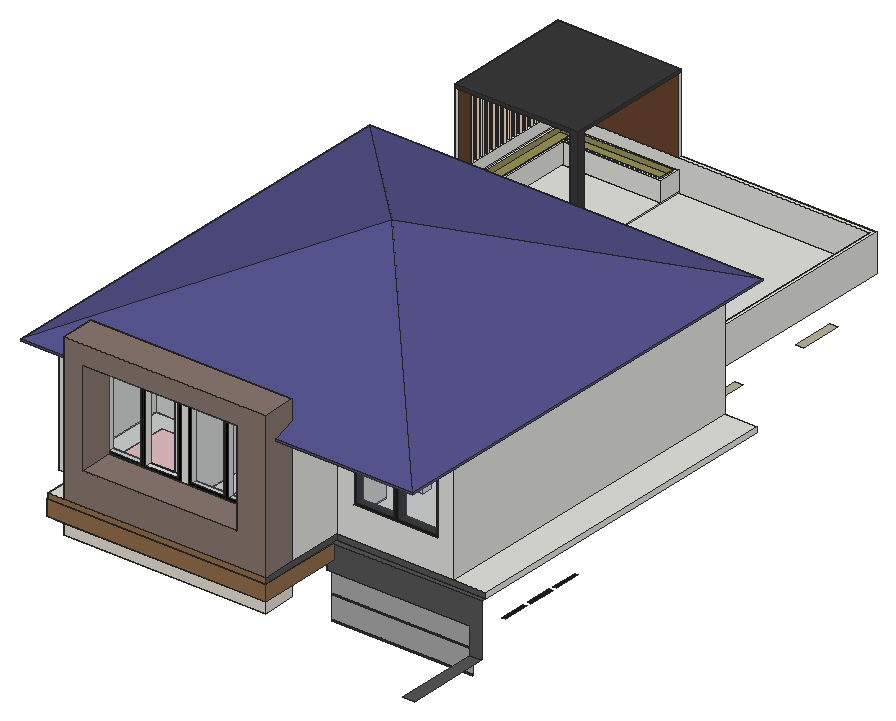
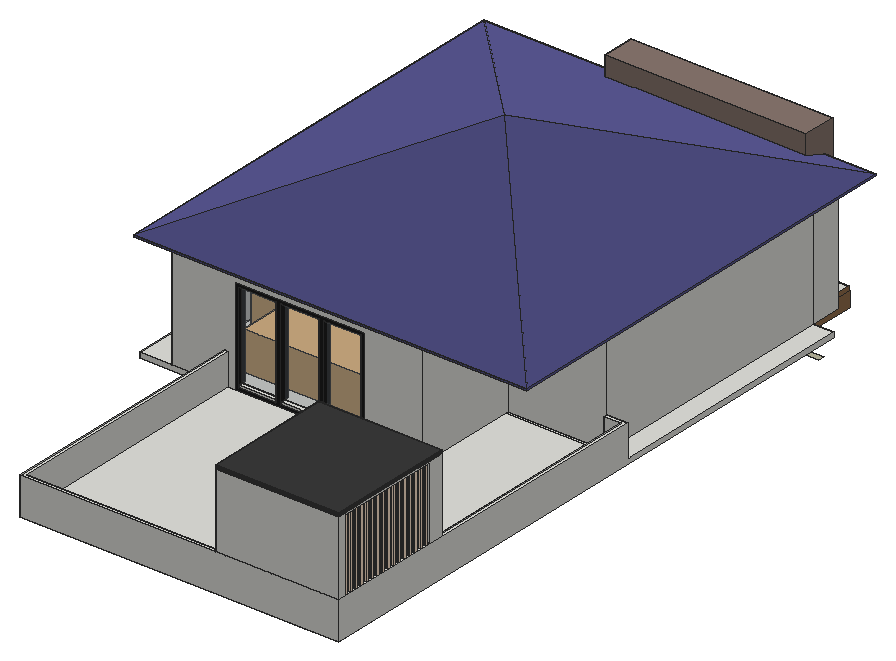
# SketchUp Ruby script. Lengths in inches.
U = 1.inch
M = Sketchup.active_model
def pt(a) = Geom::Point3d.new(a.map { |v| v * U })
def face(e, loops, mat)
  f = e.add_face(loops[0].map { |a| pt(a) })
  loops[1..].each { |l| e.add_face(l.map { |a| pt(a) }).erase! }
  f.material = f.back_material = mat if mat
  f
end
# faces: each face lists its corners as indices into pts; further lists are holes
def faces(e, pts, list, mat = nil) = list.each { |f| face(e, (f[0].is_a?(Array) ? f : [f]).map { |l| l.map { |i| pts[i] } }, mat) }
# xy, xz, yz: faces in a plane at the given z, y or x. An outline is a flat list of corners, or four numbers for a rectangle; further outlines are holes
def ring(l) = l.size == 4 ? [[l[0], l[1]], [l[2], l[1]], [l[2], l[3]], [l[0], l[3]]] : l.each_slice(2).to_a
def flat(e, list, mat, &to3) = list.each { |f| face(e, (f[0].is_a?(Array) ? f : [f]).map { |l| ring(l).map { |u, v| to3.(u, v) } }, mat) }
def xy(e, z, list, mat = nil) = flat(e, list, mat) { |x, y| [x, y, z] }
def xz(e, y, list, mat = nil) = flat(e, list, mat) { |x, z| [x, y, z] }
def yz(e, x, list, mat = nil) = flat(e, list, mat) { |y, z| [x, y, z] }
def lines(e, pts, list) = list.each { |a, b| e.add_line(pt(pts[a]), pt(pts[b])) }
# prism: a flat outline (further loops are holes) pulled along v
def prism(e, loops, v, mat = nil)
  f = face(e, loops, mat); d = Geom::Vector3d.new(v.map { |x| x * U })
  f.pushpull(f.normal.samedirection?(d) ? d.length : -d.length)
end
def box(e, o, s, mat = nil) = prism(e, [[o, [o[0] + s[0], o[1], o[2]], [o[0] + s[0], o[1] + s[1], o[2]], [o[0], o[1] + s[1], o[2]]]], [0, 0, s[2]], mat)
def at(x, y, z, deg = 0) = Geom::Transformation.translation(pt([x, y, z])) * Geom::Transformation.rotation(ORIGIN, Z_AXIS, deg.degrees)
def axes(o, x, y, z) = Geom::Transformation.new([*x, 0, *y, 0, *z, 0, *pt(o).to_a, 1])
def part(name) = M.definitions.add(name)
# library, detail: a bought-in or finely detailed component or shape, given as its bounding box
def library(name, o, s) = part(name).tap { |d| box(d.entities, o, s) }
def detail(e, o, s) = box(e.add_group.entities, o, s)
def put(e, d, t, mat = nil) = e.add_instance(d, t).tap { |i| i.material = mat if mat }
def group(e, t, mat = nil) = e.add_group.tap { |g| g.transformation = t; g.material = mat if mat }.entities
root = M.entities
M.materials.add("A01_Blush_Petal").color = [255, 204, 204]
M.materials.add("C01_Vanilla_Cream").color = [255, 230, 206]
M.materials.add("Concrete_04_1K").color = [184, 181, 156]
M.materials.add("F01_Seafoam_Drift").color = [229, 255, 204]
M.materials.add("G01_Mint_Mist").color = [204, 255, 204]
M.materials.add("Glass_Basic_01").color = [161, 173, 186]
M.materials["Glass_Basic_01"].alpha = 0.25
M.materials.add("Glass_Mirror_01").color = [185, 185, 185]
M.materials.add("L01_Cotton_Candy").color = [255, 204, 229]
M.materials.add("M03_Pewter_Shine").color = [168, 168, 168]
M.materials.add("M06_Steel_Smoke").color = [86, 86, 86]
M.materials.add("M07_Charcoal_Gleam").color = [58, 58, 58]
M.materials.add("M08_Obsidian_Black").color = [30, 30, 30]
M.materials.add("M09_Shadow_Night").color = [0, 0, 0]
M.materials.add("Marble_01_1K").color = [230, 221, 211]
M.materials.add("Metal_06_1K").color = [238, 236, 231]
M.materials.add("Plywood_08_1K").color = [202, 166, 113]
M.materials.add("Roofing_07_1K").color = [87, 85, 143]
M.materials.add("Soil_04_1K").color = [152, 146, 88]
M.materials.add("Wood_Floor_01_1K").color = [146, 111, 76]
M.materials.add("Wood_Floor_12_1K").color = [137, 119, 111]
M.materials.add("Wood_Veneer_15_1K").color = [103, 69, 45]
c1 = part("Group\#16")
box(c1.entities,[0,0,0],[9,36,9])
c2 = part("Group\#15")
box(c2.entities,[0,0,0],[9,36,9])
c3 = part("Group\#65")
detail(c3.entities,[3.98,0,0],[59.19,63.17,43.625])
c4 = library("Group\#63",[0,0,0],[138,56.37,43.625])
c5 = part("Group\#87")
prism(c5.entities,[[[12.875,15.85,0],[12.875,5.875,0],[12.54,4.32,0],[11.83,2.9,0],[10.8,1.69,0],[9.5,0.77,0],[8.02,0.2,0],[6.4375,0,0],[4.86,0.2,0],[3.375,0.77,0],[2.08,1.69,0],[1.05,2.9,0],[0.34,4.32,0],[0,5.875,0],[0,15.85,0],[0.52,17.21,0],[1.32,18.43,0],[2.37,19.44,0],[3.61,20.2,0],[4.99,20.67,0],[6.4375,20.83,0],[7.89,20.67,0],[9.27,20.2,0],[10.51,19.44,0],[11.56,18.43,0],[12.36,17.21,0]]],[0,0,2])
c6 = part("Group\#86")
xy(c6.entities,0,[[0,0,78.6875,56.125]])
xy(c6.entities,12,[[0,0,78.6875,56.125]],"A01_Blush_Petal")
xz(c6.entities,0,[[0,0,78.6875,12]],"A01_Blush_Petal")
xz(c6.entities,56.125,[[0,0,78.6875,12]],"A01_Blush_Petal")
yz(c6.entities,0,[[0,0,56.125,12]])
yz(c6.entities,78.6875,[[0,0,56.125,12]],"A01_Blush_Petal")
put(c6.entities,c5,at(5.56,5.57,12),"G01_Mint_Mist")
put(c6.entities,c5,at(5.56,28.95,12),"G01_Mint_Mist")
xy(root,81.29,[[4861.07,3566.51,4874.8125,3660.98]],"M06_Steel_Smoke")
xy(root,99,[[4550.5625,3805.79,4586.5625,3809.79],[4591.8125,3833.04,4595.8125,3869.04],[4784.8125,3923.04,4825.3125,3929.04],[4586.8125,4226.61,4591.8125,4262.61]],"Concrete_04_1K")
xy(root,105.07,[[4586.8125,3932.41,4591.3125,3997.24],[4591.3125,3932.41,4595.8125,3997.24]],"M08_Obsidian_Black")
xy(root,107.45,[[4584.8125,4077.51,4588.3125,4117.75],[4588.3125,4077.51,4591.8125,4117.75],[4584.8125,4127.84,4588.3125,4177.75],[4588.3125,4127.84,4591.8125,4177.75]],"M08_Obsidian_Black")
xy(root,108,[[4870.8125,3694.73,4874.8125,3724.73],[4870.8125,3730.73,4874.8125,3760.73],[4870.8125,3766.73,4874.8125,3796.73],[4492.8125,4193.04,4518.8125,4197.54],[4520.8125,4193.04,4546.8125,4197.54]],"M08_Obsidian_Black")
xy(root,111,[[4498.625,3604.45,4546.625,3606.54],[4553.37,3604.45,4601.37,3608.64],[4498.625,3606.54,4546.625,3608.64],[4634.06,3666.98,4682.06,3670.98],[4769.8125,4101.42,4778.8125,4149.42],
  [4489.8125,4193.04,4549.8125,4197.54],[4489.8125,4197.54,4549.8125,4202.04],[4769.8125,4234.61,4778.8125,4282.61]],"Concrete_04_1K")
xy(root,111,[[4700.3125,3660.98,4861.07,3666.98]],"M06_Steel_Smoke")
xy(root,111,[[4584.8125,4073.96,4586.8125,4121.29],[4584.8125,4124.29,4586.8125,4181.29]],"M08_Obsidian_Black")
xy(root,117.5625,[[4432.07,3639.11,4462.07,3645.11]],"Concrete_04_1K")
xy(root,124.125,[[4462.07,3564.51,4480,3639.11]],"Concrete_04_1K")
xy(root,124.125,[[4480,3564.51,4480,3604.45,4700.3125,3604.45,4700.3125,3660.98,4708.6875,3660.98,4708.6875,3564.51]],"Plywood_08_1K")
xy(root,141,[[[4480,3604.45,4625.87,3604.45,4625.87,3666.98,4695.7,3666.98,4695.7,3604.45,4700.3125,3604.45,4700.3125,3666.98,4874.8125,3666.98,4874.8125,3833.04,4870.8125,3833.04,4870.8125,3670.98,4690.8125,3670.98,4690.8125,3833.04,4686.8125,3833.04,4686.8125,3670.98,4625.87,3670.98,4625.87,3750.01,4595.8125,3750.01,4595.8125,3878.04,4480,3878.04,4480,3809.79,4420.38,3809.79,4420.38,3639.11,4480,3639.11],[4489,3608.64,4489,3805.79,4591.8125,3805.79,4591.8125,3746.01,4621.87,3746.01,4621.87,3608.64],[4429.38,3645.11,4480,3800.79],[4489,3809.79,4591.8125,3869.04]],[4646.8125,3770.04,4650.8125,3770.04,4650.8125,3869.04,4741.125,3869.04,4741.125,3878.04,4646.8125,3878.04],[4690.8125,3829.04,4741.125,3833.04],[4777.125,3829.04,4870.8125,3833.04],[[4865.8125,3833.04,4874.8125,3833.04,4874.8125,4049.04,4778.8125,4049.04,4778.8125,4337.04,4454.8125,4337.04,4454.8125,4193.04,4586.8125,4193.04,4586.8125,4058.04,4480,4058.04,4480,4049.04,4591.8125,4049.04,4591.8125,4328.04,4769.8125,4328.04,4769.8125,4040.04,4865.8125,4040.04,4865.8125,3983.04,4784.8125,3983.04,4784.8125,4010.04,4778.8125,4010.04,4778.8125,3869.04,4784.8125,3869.04,4784.8125,3923.04,4825.3125,3923.04,4825.3125,3929.04,4784.8125,3929.04,4784.8125,3977.04,4865.8125,3977.04,4865.8125,3929.04,4825.3125,3929.04,4825.3125,3923.04,4865.8125,3923.04],[4463.8125,4202.04,4586.8125,4328.04]],
  [4586.8125,3878.04,4595.8125,4049.04],[4708.76,3915.92,4736.64,3915.92,4736.64,4049.04,4708.76,4049.04,4708.76,4045.04,4732.01,4045.04,4732.01,3919.92,4708.76,3919.92]],"Concrete_04_1K")
xy(root,141,[[4700.3125,3604.45,4708.6875,3604.45,4708.6875,3660.98,4874.8125,3660.98,4874.8125,3666.98,4700.3125,3666.98]],"M06_Steel_Smoke")
xy(root,141.1875,[[4462.07,3564.51,4708.6875,3564.51,4708.6875,3604.45,4480,3604.45,4480,3639.11,4462.07,3639.11]],"Wood_Floor_01_1K")
xy(root,153,[[4612.42,3619.02,4666.3,3697.33],[4489.57,3621.3125,4540.88,3691.6875]])
xz(root,3564.51,[[4462.07,124.125,4708.6875,141.1875]],"Wood_Floor_01_1K")
xz(root,3604.45,[[4480,124.125,4625.87,141],[4625.87,124.125,4695.7,141],[4695.7,124.125,4700.3125,141],[4480,141,4700.3125,141.1875],[4700.3125,141,4708.6875,141.1875]],"Concrete_04_1K")
xz(root,3639.11,[[4462.07,124.125,4480,141],[4462.07,141,4480,141.1875]],"Concrete_04_1K")
xz(root,3660.98,[[4861.07,81.29,4874.8125,81.29,4874.8125,141,4708.6875,141,4708.6875,124.125,4700.3125,124.125,4700.3125,111,4861.07,111]],"M06_Steel_Smoke")
xz(root,3666.98,[[4701.3125,60,4860.07,84],[4701.3125,86,4860.07,110]],"M03_Pewter_Shine")
xz(root,3666.98,[[4701.3125,58,4860.07,60],[4701.3125,84,4860.07,86]],"M07_Charcoal_Gleam")
xz(root,3923.04,[[4784.8125,99,4825.3125,141]],"M03_Pewter_Shine")
xz(root,3929.04,[[4784.8125,99,4825.3125,141]],"L01_Cotton_Candy")
yz(root,4462.07,[[3564.51,124.125,3639.11,141.1875]],"Wood_Floor_01_1K")
yz(root,4480,[[3604.45,124.125,3639.11,141],[3604.45,141,3639.11,141.1875]],"Concrete_04_1K")
yz(root,4591.8125,[[3833.04,99,3869.04,141]],"L01_Cotton_Candy")
yz(root,4595.8125,[[3833.04,99,3869.04,141]],"L01_Cotton_Candy")
yz(root,4700.3125,[[3660.98,111,3666.98,111,3666.98,141,3604.45,141,3604.45,124.125,3660.98,124.125]],"Concrete_04_1K")
yz(root,4708.6875,[[3564.51,124.125,3660.98,124.125,3660.98,141,3604.45,141,3604.45,141.1875,3564.51,141.1875]],"Wood_Floor_01_1K")
g1 = group(root,at(4578.37,3805.79,56.68))
prism(g1,[[[1.19,0,3.08],[1.59,0,3.125],[1.99,0,3.0625],[2.37,0,2.9],[2.6875,0,2.65],[2.93,0,2.32],[3.08,0,1.9375],[3.125,0,1.53],[3.0625,0,1.13],[2.9,0,0.76],[2.65,0,0.4375],[2.32,0,0.2],[1.9375,0,0.05],[1.53,0,0],[1.13,0,0.0625],[0.76,0,0.22],[0.4375,0,0.48],[0.2,0,0.81],[0.05,0,1.19],[0,0,1.59],[0.0625,0,1.99],[0.22,0,2.37],[0.48,0,2.6875],[0.81,0,2.93]]],[0,-0.4375,0],"Metal_06_1K")
g2 = group(root,at(4521.09,3785.04,69.49))
prism(g2,[[[1.39,0,3.6875],[1.875,0,3.75],[2.36,0,3.6875],[2.8125,0,3.5],[3.2,0,3.2],[3.5,0,2.8125],[3.6875,0,2.36],[3.75,0,1.875],[3.6875,0,1.39],[3.5,0,0.9375],[3.2,0,0.55],[2.8125,0,0.25],[2.36,0,0.0625],[1.875,0,0],[1.39,0,0.0625],[0.9375,0,0.25],[0.55,0,0.55],[0.25,0,0.9375],[0.0625,0,1.39],[0,0,1.875],[0.0625,0,2.36],[0.25,0,2.8125],[0.55,0,3.2],[0.9375,0,3.5]]],[0,-1,0],"Metal_06_1K")
g3 = group(root,at(4480,3604.45,111))
box(g3,[0,-37.9375,0],[226.6875,37.9375,13.125],"Marble_01_1K")
g4 = group(root,at(4443.375,3604.44,141))
xy(g4,0,[[234.125,264.6,240.125,273.6],[240.125,264.6,289.8125,273.6]])
xy(g4,6,[[161.8125,165.6,197.8125,174.6],[161.8125,174.6,197.8125,183.6],[161.8125,183.6,197.8125,192.6],[161.8125,192.6,197.8125,201.6],[161.8125,201.6,197.8125,210.6],
  [161.8125,210.6,197.8125,219.6],[161.8125,219.6,197.8125,228.6],[161.8125,228.6,197.8125,264.6],[197.8125,228.6,207.125,264.6],[207.125,228.6,216.125,264.6],
  [216.125,228.6,225.125,264.6],[225.125,228.6,234.125,264.6],[234.125,228.6,243.125,264.6],[243.125,228.6,252.125,264.6],[252.125,228.6,289.8125,264.6]])
xz(g4,228.6,[[197.8125,0,201.8125,6],[201.8125,0,289.8125,6]])
xz(g4,264.6,[[234.125,0,240.125,6],[240.125,0,289.8125,6]])
xz(g4,273.6,[[234.125,0,240.125,6],[240.125,0,289.8125,6]])
yz(g4,289.8125,[[228.6,0,264.6,6],[264.6,0,273.6,6]])
g5 = group(g4,at(0,0,6))
xy(g5,0,[[[0,0,0,325.35,111.8125,325.35,111.8125,444.6,394.8125,444.6,394.8125,62.54,263.3125,62.54,263.3125,0],[9,6,125.66,6,125.66,132,218.3125,132,218.3125,126,131.66,126,131.66,6,254.3125,6,254.3125,132,263.3125,132,263.3125,71.54,385.8125,71.54,385.8125,435.6,174.8125,435.6,174.8125,393.6,120.8125,393.6,120.8125,196.35,111.8125,196.35,111.8125,316.35,9,316.35,9,205.35,75.8125,205.35,75.8125,188.61,69.8125,188.61,69.8125,196.35,9,196.35,9,132,69.8125,132,69.8125,158.61,75.8125,158.61,75.8125,132,89.66,132,89.66,126,9,126],[120.8125,399.6,168.8125,435.6]]])
xy(g5,3,[[181.875,435.6,223.67,444.6],[229.67,435.6,271.875,444.6],[277.875,435.6,319.875,444.6]])
xy(g5,6,[[9,6,125.66,126],[131.66,6,254.3125,126],[[263.3125,71.54,385.8125,71.54,385.8125,435.6,319.875,435.6,319.875,440.1,277.875,440.1,277.875,435.6,271.875,435.6,271.875,440.1,229.67,440.1,229.67,435.6,223.67,435.6,223.67,440.1,181.875,440.1,181.875,435.6,174.8125,435.6,174.8125,393.6,120.8125,393.6,120.8125,196.35,75.8125,196.35,75.8125,132,263.3125,132],[197.8125,158.6,197.8125,165.6,157.8125,165.6,157.8125,268.6,234.125,268.6,234.125,273.6,289.8125,273.6,289.8125,228.6,283.8125,228.6,283.8125,199.98,277.8125,199.98,277.8125,169.98,283.8125,169.98,283.8125,158.6]],[89.66,126,125.66,132],[218.3125,126,254.3125,132],
  [9,132,69.8125,196.35],[69.8125,158.61,75.8125,188.61],[197.8125,164.6,197.8125,228.6,283.8125,228.6,283.8125,222.6,203.8125,222.6,203.8125,164.6],[203.8125,164.6,277.8125,222.6],[157.8125,165.6,161.8125,268.6],
  [161.8125,165.6,197.8125,174.6],[161.8125,174.6,197.8125,183.6],[161.8125,183.6,197.8125,192.6],[161.8125,192.6,197.8125,201.6],[75.8125,196.35,111.8125,205.35],
  [161.8125,201.6,197.8125,210.6],[9,205.35,111.8125,316.35],[161.8125,210.6,197.8125,219.6],[161.8125,219.6,197.8125,228.6],[161.8125,228.6,197.8125,264.6],
  [197.8125,228.6,207.125,264.6],[207.125,228.6,216.125,264.6],[216.125,228.6,225.125,264.6],[225.125,228.6,234.125,264.6],[234.125,228.6,243.125,264.6],
  [252.125,228.6,289.8125,264.6],[120.8125,399.6,168.8125,435.6],[223.67,435.6,229.67,440.1],[271.875,435.6,277.875,440.1],[181.875,440.1,223.67,444.6],
  [229.67,440.1,271.875,444.6],[277.875,440.1,319.875,444.6]])
xy(g5,39,[[20.75,0,50.75,6],[56.75,0,92.75,6],[98.75,0,134.75,6],[149.625,0,185.625,6],[191.625,0,227.625,6]])
xy(g5,39,[[285.75,62.54,327.75,71.54],[333.75,62.54,375.75,71.54]],"M08_Obsidian_Black")
xy(g5,90,[[277.8125,169.98,283.8125,199.98]])
xy(g5,105,[[181.875,435.6,223.67,440.1],[229.67,435.6,271.875,440.1],[277.875,435.6,319.875,440.1],[181.875,440.1,223.67,444.6],[229.67,440.1,271.875,444.6],
  [277.875,440.1,319.875,444.6]])
xy(g5,126.25,[[20.75,0,50.75,6],[56.75,0,92.75,6],[98.75,0,134.75,6],[149.625,0,185.625,6],[191.625,0,227.625,6]])
xy(g5,126.6875,[[285.75,62.54,327.75,71.54],[333.75,62.54,375.75,71.54]],"M08_Obsidian_Black")
xy(g5,132,[[[0,0,263.3125,0,263.3125,62.54,394.8125,62.54,394.8125,444.6,111.8125,444.6,111.8125,325.35,0,325.35],[9,6,9,126,89.66,126,89.66,132,75.8125,132,75.8125,158.61,69.8125,158.61,69.8125,132,9,132,9,196.35,69.8125,196.35,69.8125,188.61,75.8125,188.61,75.8125,205.35,9,205.35,9,316.35,111.8125,316.35,111.8125,196.35,120.8125,196.35,120.8125,393.6,174.8125,393.6,174.8125,435.6,385.8125,435.6,385.8125,71.54,263.3125,71.54,263.3125,132,254.3125,132,254.3125,6,131.66,6,131.66,126,218.3125,126,218.3125,132,125.66,132,125.66,6],[120.8125,399.6,168.8125,435.6]],[197.8125,158.6,283.8125,158.6,283.8125,222.6,277.8125,222.6,277.8125,164.6,197.8125,164.6],[197.8125,164.6,203.8125,164.6,203.8125,222.6,283.8125,222.6,283.8125,228.6,197.8125,228.6]])
xy(g5,133.875,[[157.8125,165.6,161.8125,268.6],[161.8125,264.6,289.8125,264.6,289.8125,273.6,234.125,273.6,234.125,268.6,161.8125,268.6]])
xz(g5,0,[[[0,0,263.3125,132],[17.75,36,137.75,129.25],[146.625,36,230.625,129.25]]])
xz(g5,0,[[20.75,39,50.75,126.25],[56.75,39,92.75,126.25],[149.625,39,185.625,126.25],[191.625,39,227.625,126.25]],"Glass_Basic_01")
xz(g5,0,[[[17.75,36,53.75,129.25],[20.75,39,50.75,126.25]],[[53.75,36,95.75,129.25],[56.75,39,92.75,126.25]],[[95.75,36,137.75,129.25],[98.75,39,134.75,126.25]],[[146.625,36,188.625,129.25],[149.625,39,185.625,126.25]],[[188.625,36,230.625,129.25],[191.625,39,227.625,126.25]]],"M09_Shadow_Night")
xz(g5,6,[[9,0,125.66,6],[131.66,0,254.3125,6],[[9,6,9,132,125.66,132,125.66,126.25,98.75,126.25,98.75,39,125.66,39,125.66,6],[56.75,39,92.75,126.25],[20.75,39,50.75,126.25]],[[131.66,6,131.66,39,134.75,39,134.75,126.25,131.66,126.25,131.66,132,254.3125,132,254.3125,6],[149.625,39,185.625,126.25],[191.625,39,227.625,126.25]],[125.66,39,131.66,126.25],
  [131.66,39,134.75,126.25]])
xz(g5,6,[[98.75,39,125.66,126.25]],"Glass_Basic_01")
xz(g5,62.54,[[[263.3125,0,394.8125,132],[282.75,36,378.75,129.6875]]])
xz(g5,62.54,[[[282.75,36,378.75,129.6875],[285.75,39,327.75,126.6875],[333.75,39,375.75,126.6875]]],"M08_Obsidian_Black")
xz(g5,71.54,[[263.3125,0,385.8125,6],[[263.3125,6,385.8125,132],[285.75,39,327.75,126.6875],[333.75,39,375.75,126.6875]]])
xz(g5,126,[[9,0,89.66,6],[131.66,0,218.3125,6],[9,6,89.66,132],[131.66,6,218.3125,132]])
xz(g5,132,[[9,0,69.8125,6],[75.8125,0,81,6],[81,0,87,6],[87,0,89.66,6],[125.66,0,218.3125,6],
  [254.3125,0,263.3125,6],[9,6,69.8125,132],[75.8125,6,81,132],[81,6,87,132],[87,6,89.66,132],
  [125.66,6,218.3125,132],[254.3125,6,263.3125,132]])
xz(g5,158.6,[[197.8125,6,283.8125,132]])
xz(g5,158.61,[[69.8125,0,75.8125,6],[69.8125,6,75.8125,132]])
xz(g5,164.6,[[197.8125,6,203.8125,132],[203.8125,6,277.8125,132]])
xz(g5,165.6,[[157.8125,6,161.8125,133.875]])
xz(g5,169.98,[[277.8125,6,283.8125,90]])
xz(g5,188.61,[[69.8125,0,75.8125,6],[69.8125,6,75.8125,132]])
xz(g5,196.35,[[9,0,69.8125,6],[111.8125,0,120.8125,6],[9,6,69.8125,132],[111.8125,6,120.8125,132]])
xz(g5,199.98,[[277.8125,6,283.8125,90]])
xz(g5,205.35,[[9,0,75.8125,6],[9,6,75.8125,132]])
xz(g5,222.6,[[203.8125,6,277.8125,132],[277.8125,6,283.8125,132]])
xz(g5,228.6,[[197.8125,6,283.8125,132]])
xz(g5,264.6,[[161.8125,6,243.125,133.875],[243.125,6,252.125,133.875],[252.125,6,289.8125,133.875]])
xz(g5,268.6,[[157.8125,6,161.8125,133.875],[161.8125,6,234.125,133.875]])
xz(g5,273.6,[[234.125,6,289.8125,133.875]])
xz(g5,316.35,[[9,0,111.8125,6],[9,6,111.8125,132]])
xz(g5,325.35,[[0,0,111.8125,132]])
xz(g5,393.6,[[120.8125,0,174.8125,6],[120.8125,6,174.8125,132]])
xz(g5,399.6,[[120.8125,0,168.8125,6],[120.8125,6,168.8125,132]])
xz(g5,435.6,[[120.8125,0,168.8125,6],[174.8125,0,385.8125,0,385.8125,6,319.875,6,319.875,3,277.875,3,277.875,6,271.875,6,271.875,3,229.67,3,229.67,6,223.67,6,223.67,3,181.875,3,181.875,6,174.8125,6],[120.8125,6,168.8125,132],[174.8125,6,181.875,6,181.875,105,223.67,105,223.67,6,229.67,6,229.67,105,271.875,105,271.875,6,277.875,6,277.875,105,319.875,105,319.875,6,385.8125,6,385.8125,132,174.8125,132]])
xz(g5,444.6,[[111.8125,0,111.8125,132,394.8125,132,394.8125,0,322.875,0,322.875,108,178.875,108,178.875,0],[181.875,3,223.67,6],[229.67,3,271.875,6],[277.875,3,319.875,6]])
xz(g5,444.6,[[[178.875,0,322.875,108],[229.67,3,271.875,105],[277.875,3,319.875,105],[181.875,3,223.67,105]]],"M08_Obsidian_Black")
yz(g5,0,[[0,0,34.67,132],[34.67,0,325.35,132]])
yz(g5,9,[[6,0,126,6],[132,0,196.35,6],[205.35,0,316.35,6],[6,6,126,132],[132,6,196.35,132],
  [205.35,6,316.35,132]])
yz(g5,20.75,[[0,39,6,126.25]])
yz(g5,50.75,[[0,39,6,126.25]])
yz(g5,56.75,[[0,39,6,126.25]])
yz(g5,69.8125,[[132,0,158.61,6],[188.61,0,196.35,6],[132,6,158.61,132],[188.61,6,196.35,132]])
yz(g5,75.8125,[[132,0,158.61,6],[188.61,0,196.35,6],[196.35,0,205.35,6],[132,6,158.61,132],[188.61,6,196.35,132],
  [196.35,6,205.35,132]])
yz(g5,89.66,[[126,0,132,6],[126,6,132,132]])
yz(g5,92.75,[[0,39,6,126.25]])
yz(g5,98.75,[[0,39,6,126.25]])
yz(g5,111.8125,[[196.35,0,205.35,6],[205.35,0,316.35,6],[325.35,0,444.6,132],[196.35,6,205.35,132],[205.35,6,316.35,132]])
yz(g5,120.8125,[[196.35,0,393.6,6],[399.6,0,435.6,6],[196.35,6,393.6,132],[399.6,6,435.6,132]])
yz(g5,125.66,[[6,0,126,6],[126,0,132,6],[6,6,126,132],[126,6,132,132]])
yz(g5,131.66,[[6,0,126,6],[6,6,126,132]])
yz(g5,134.75,[[0,39,6,126.25]])
yz(g5,149.625,[[0,39,6,126.25]])
yz(g5,157.8125,[[165.6,6,268.6,133.875]])
yz(g5,161.8125,[[165.6,6,264.6,133.875],[264.6,6,268.6,133.875]])
yz(g5,168.8125,[[399.6,0,435.6,6],[399.6,6,435.6,132]])
yz(g5,174.8125,[[393.6,0,435.6,6],[393.6,6,435.6,132]])
yz(g5,181.875,[[435.6,3,444.6,6]])
yz(g5,181.875,[[435.6,6,440.1,105],[440.1,6,444.6,105]],"M08_Obsidian_Black")
yz(g5,185.625,[[0,39,6,126.25]])
yz(g5,191.625,[[0,39,6,126.25]])
yz(g5,197.8125,[[158.6,6,164.6,132],[164.6,6,174.6,132],[174.6,6,228.6,132]])
yz(g5,203.8125,[[164.6,6,222.6,132]])
yz(g5,218.3125,[[126,0,132,6],[126,6,132,132]])
yz(g5,223.67,[[435.6,3,444.6,6]])
yz(g5,223.67,[[435.6,6,444.6,105]],"M08_Obsidian_Black")
yz(g5,227.625,[[0,39,6,126.25]])
yz(g5,229.67,[[435.6,3,444.6,6]])
yz(g5,229.67,[[435.6,6,444.6,105]],"M08_Obsidian_Black")
yz(g5,234.125,[[268.6,6,273.6,133.875]])
yz(g5,254.3125,[[6,0,126,6],[126,0,132,6],[6,6,126,132],[126,6,132,132]])
yz(g5,263.3125,[[0,0,62.54,132],[71.54,0,132,6],[71.54,6,132,132]])
yz(g5,271.875,[[435.6,3,444.6,6]])
yz(g5,271.875,[[435.6,6,444.6,105]],"M08_Obsidian_Black")
yz(g5,277.8125,[[164.6,6,164.6,132,222.6,132,222.6,6,199.98,6,199.98,90,169.98,90,169.98,6]])
yz(g5,277.875,[[435.6,3,444.6,6]])
yz(g5,277.875,[[435.6,6,444.6,105]],"M08_Obsidian_Black")
yz(g5,283.8125,[[158.6,6,169.98,6,169.98,90,199.98,90,199.98,6,222.6,6,222.6,132,158.6,132],[222.6,6,228.6,132]])
yz(g5,285.75,[[62.54,39,71.54,126.6875]],"M08_Obsidian_Black")
yz(g5,289.8125,[[264.6,6,273.6,133.875]])
yz(g5,319.875,[[435.6,3,444.6,6]])
yz(g5,319.875,[[435.6,6,440.1,105],[440.1,6,444.6,105]],"M08_Obsidian_Black")
yz(g5,327.75,[[62.54,39,71.54,126.6875]],"M08_Obsidian_Black")
yz(g5,333.75,[[62.54,39,71.54,126.6875]],"M08_Obsidian_Black")
yz(g5,375.75,[[62.54,39,71.54,126.6875]],"M08_Obsidian_Black")
yz(g5,385.8125,[[71.54,0,435.6,6],[71.54,6,435.6,132]])
yz(g5,394.8125,[[62.54,0,444.6,132]])
p = [[197.8125,165.6,0],[197.8125,152.6,0],[265.625,152.6,0],[289.8125,152.6,0],[289.8125,228.6,0],[289.8125,191.84,0],
  [234.125,268.6,0],[157.8125,268.6,0],[157.8125,165.6,0],[161.8125,165.6,0],[289.8125,161.84,0],[283.8125,161.84,0],
  [283.8125,191.84,0]]
lines(g5,p,[[0,1],[1,2],[2,3],[4,5],[6,7],[7,8],[9,8],[10,3],[11,10],[5,10],[12,5]])
put(g5,c1,at(243.125,228.6,6))
put(g5,c1,at(234.125,228.6,15))
put(g5,c1,at(225.125,228.6,24))
put(g5,c1,at(216.125,228.6,33))
put(g5,c1,at(207.125,228.6,42))
put(g5,c1,at(198.125,228.6,51))
g6 = group(g5,at(189.125,228.6,60))
box(g6,[-27.3125,0,0],[36.3125,36,9])
put(g5,c2,at(198.125,219.6,69,90))
put(g5,c2,at(198.125,210.6,78,90))
put(g5,c2,at(198.125,201.6,87,90))
put(g5,c2,at(198.125,192.6,96,90))
put(g5,c2,at(198.125,183.6,105,90))
put(g5,c2,at(198.125,174.6,114,90))
put(g5,c2,at(198.125,165.6,123,90))
g7 = group(g5,at(181.875,440.1,6),"Glass_Basic_01")
xz(g7,0,[[0,0,138,99]])
g8 = group(root,at(4454.8125,3666.98,141))
xy(g8,0,[[7.26,-100.47,7.26,-27.875,-34.43,-27.875,-34.43,670.0625,324,670.0625,324,382.0625,420,382.0625,420,0,251.875,0,251.875,-100.47]])
xy(g8,6,[[7.26,-100.47,251.875,-100.47,251.875,0,420,0,420,382.0625,320,382.0625,320,666.0625,-30.43,666.0625,-30.43,266.8125,100.375,266.8125,100.375,262.8125,-34.43,262.8125,-34.43,-27.875,7.26,-27.875],[-11.4375,262.8125,100.375,266.8125]])
xy(g8,42,[[-34.43,262.8125,-11.4375,262.8125,-11.4375,266.8125,-30.43,266.8125,-30.43,524.58,-34.43,524.58],[320,382.0625,324,382.0625,324,670.0625,104.06,670.0625,104.06,666.0625,320,666.0625],[-34.43,524.58,-30.43,540.68],[-34.43,540.68,-30.43,661.0625],[-34.43,661.0625,-34.43,670.0625,104.06,670.0625,104.06,666.0625,-30.43,666.0625,-30.43,661.0625]])
xy(g8,123.57,[[-34.43,540.68,-30.43,661.0625]])
xy(g8,126,[[-34.43,524.58,-30.43,666.0625],[-34.43,666.0625,104.06,670.0625]])
xz(g8,-100.47,[[7.26,0,251.875,6]],"Wood_Floor_01_1K")
xz(g8,-27.875,[[-34.43,0,7.26,6]])
xz(g8,0,[[251.875,0,420,6]],"M06_Steel_Smoke")
xz(g8,262.8125,[[-34.43,6,-11.4375,42]])
xz(g8,266.8125,[[-30.43,6,-11.4375,42]])
xz(g8,382.0625,[[324,0,420,6],[320,6,324,42]])
xz(g8,524.58,[[-34.43,42,-30.43,126]])
xz(g8,540.68,[[-34.43,42,-30.43,123.57]])
xz(g8,661.0625,[[-34.43,42,-30.43,123.57]])
xz(g8,666.0625,[[-30.43,6,320,42]])
xz(g8,666.0625,[[-30.43,42,104.06,126]],"Wood_Veneer_15_1K")
xz(g8,670.0625,[[-34.43,0,324,42],[-34.43,42,104.06,126]])
yz(g8,-34.43,[[-27.875,0,-27.875,6,262.8125,6,262.8125,42,670.0625,42,670.0625,0],[524.58,42,524.58,126,670.0625,126,670.0625,42,661.0625,42,661.0625,123.57,540.68,123.57,540.68,42]])
yz(g8,-30.43,[[266.8125,6,666.0625,42]])
yz(g8,-30.43,[[524.58,42,540.68,42,540.68,123.57,661.0625,123.57,661.0625,42,666.0625,42,666.0625,126,524.58,126]],"Wood_Veneer_15_1K")
yz(g8,-11.4375,[[262.8125,6,266.8125,42]])
yz(g8,7.26,[[-100.47,0,-27.875,6]],"Wood_Floor_01_1K")
yz(g8,104.06,[[666.0625,42,670.0625,126]])
yz(g8,251.875,[[-100.47,0,0,6]],"M06_Steel_Smoke")
yz(g8,320,[[382.0625,6,666.0625,42]])
yz(g8,324,[[382.0625,0,670.0625,42]])
yz(g8,420,[[0,0,382.0625,6]])
p = [[0,526.0625,0],[-34.43,526.0625,0]]
lines(g8,p,[[0,1]])
g9 = group(g8,at(-30.43,524.58,6))
box(g9,[0,0,0],[134.49,141.49,1])
g10 = group(g8,at(-30.43,524.58,126),"M07_Charcoal_Gleam")
xy(g10,-120,[[125.49,0,134.49,9]])
xy(g10,0,[[-4,0,-4,145.49,134.49,145.49,134.49,9,125.49,9,125.49,0]])
xy(g10,4,[[-4,0,134.49,145.49]])
xz(g10,0,[[125.49,-120,134.49,-120,134.49,4,-4,4,-4,0,125.49,0]])
xz(g10,9,[[125.49,-120,134.49,0]])
xz(g10,145.49,[[-4,0,134.49,4]])
yz(g10,-4,[[0,0,145.49,4]])
yz(g10,125.49,[[0,-120,9,0]])
yz(g10,134.49,[[0,-120,9,-120,9,0,145.49,0,145.49,4,0,4]])
g11 = group(g8,at(-33.85,658.08,42),"C01_Vanilla_Cream")
box(g11,[0,0,0],[2.5,2,83.0625])
g12 = group(g8,at(-33.85,650.48,42),"C01_Vanilla_Cream")
box(g12,[0,0,0],[2.5,2,83.0625])
g13 = group(g8,at(-33.85,642.88,42),"C01_Vanilla_Cream")
box(g13,[0,0,0],[2.5,2,83.0625])
g14 = group(g8,at(-33.85,635.29,42),"C01_Vanilla_Cream")
box(g14,[0,0,0],[2.5,2,83.0625])
g15 = group(g8,at(-33.85,627.69,42),"C01_Vanilla_Cream")
box(g15,[0,0,0],[2.5,2,83.0625])
g16 = group(g8,at(-33.85,620.1,42),"C01_Vanilla_Cream")
box(g16,[0,0,0],[2.5,2,83.0625])
g17 = group(g8,at(-33.85,612.5,42),"C01_Vanilla_Cream")
box(g17,[0,0,0],[2.5,2,83.0625])
g18 = group(g8,at(-33.85,604.91,42),"C01_Vanilla_Cream")
box(g18,[0,0,0],[2.5,2,83.0625])
g19 = group(g8,at(-33.85,597.31,42),"C01_Vanilla_Cream")
box(g19,[0,0,0],[2.5,2,83.0625])
g20 = group(g8,at(-33.85,589.71,42),"C01_Vanilla_Cream")
box(g20,[0,0,0],[2.5,2,83.0625])
g21 = group(g8,at(-33.85,582.12,42),"C01_Vanilla_Cream")
box(g21,[0,0,0],[2.5,2,83.0625])
g22 = group(g8,at(-33.85,574.52,42),"C01_Vanilla_Cream")
box(g22,[0,0,0],[2.5,2,81.0625])
g23 = group(g8,at(-33.85,566.93,42),"C01_Vanilla_Cream")
box(g23,[0,0,0],[2.5,2,83])
g24 = group(g8,at(-33.85,559.33,42),"C01_Vanilla_Cream")
box(g24,[0,0,0],[2.5,2,83])
g25 = group(g8,at(-33.85,551.73,42),"C01_Vanilla_Cream")
box(g25,[0,0,0],[2.5,2,83.5625])
g26 = group(g8,at(-33.85,544.14,42),"C01_Vanilla_Cream")
box(g26,[0,0,0],[2.5,2,82.25])
g27 = group(g8,at(-30.43,527.75,7))
xy(g27,0,[[0,0,24,138.3125]])
xy(g27,16.375,[[3,3,21,135.3125]],"Soil_04_1K")
xy(g27,22.375,[[[0,0,24,138.3125],[3,3,21,135.3125]]])
xz(g27,0,[[0,0,24,22.375]])
xz(g27,3,[[3,16.375,21,22.375]],"Soil_04_1K")
xz(g27,135.3125,[[3,16.375,21,22.375]],"Soil_04_1K")
xz(g27,138.3125,[[0,0,24,22.375]])
yz(g27,0,[[0,0,138.3125,22.375]])
yz(g27,3,[[3,16.375,135.3125,22.375]],"Soil_04_1K")
yz(g27,21,[[3,16.375,135.3125,22.375]],"Soil_04_1K")
yz(g27,24,[[0,0,138.3125,22.375]])
g28 = group(g8,at(-6.43,641.25,7))
xy(g28,0,[[[0,0,110.49,24.8125],[3,3,107.49,21.8125]]])
xy(g28,16.375,[[3,3,107.49,21.8125]],"Soil_04_1K")
xy(g28,22.375,[[[0,0,110.49,24.8125],[3,3,107.49,21.8125]]])
xz(g28,0,[[0,0,110.49,22.375]])
xz(g28,3,[[3,16.375,107.49,22.375]],"Soil_04_1K")
xz(g28,21.8125,[[3,16.375,107.49,22.375]],"Soil_04_1K")
xz(g28,24.8125,[[0,0,110.49,22.375]])
yz(g28,0,[[0,0,24.8125,22.375]])
yz(g28,3,[[3,16.375,21.8125,22.375]],"Soil_04_1K")
yz(g28,107.49,[[3,16.375,21.8125,22.375]],"Soil_04_1K")
yz(g28,110.49,[[0,0,24.8125,22.375]])
p = [[3,21.8125,0],[3,21.8125,16.375],[107.49,21.8125,0],[107.49,21.8125,16.375],[3,3,0],[3,3,16.375],
  [107.49,3,0],[107.49,3,16.375]]
lines(g28,p,[[0,1],[2,3],[4,5],[6,7]])
g29 = group(root,at(4490.34,3566.51,147),"Wood_Floor_12_1K")
xy(g29,0,[[-10.875,0,216.35,37.93]])
xy(g29,36,[[10.07,0,183.66,37.93]])
xy(g29,142.81,[[10.07,0,183.66,37.93]])
xy(g29,163.8125,[[-10.875,0,216.35,37.93]])
xz(g29,0,[[[-10.875,0,216.35,163.8125],[10.07,36,183.66,142.81]]])
xz(g29,37.93,[[-10.875,0,-10.875,163.8125,10.07,163.8125,10.07,36,183.66,36,183.66,142.81,10.07,142.81,10.07,163.8125,216.35,163.8125,216.35,0]])
yz(g29,-10.875,[[0,0,37.93,163.8125]])
yz(g29,10.07,[[0,36,37.93,142.81]])
yz(g29,183.66,[[0,36,37.93,142.81]])
yz(g29,216.35,[[0,0,37.93,163.8125]])
put(root,c3,at(4753.82,3901.09,153),"F01_Seafoam_Drift")
put(root,c4,at(4636.44,3971.15,153),"F01_Seafoam_Drift")
put(root,c6,at(4458.24,3826.74,153))
put(root,c6,at(4544.16,3615.55,153,90))
put(root,c3,at(4650.08,3970.23,153,180),"F01_Seafoam_Drift")
put(root,c6,at(4667.2,3622.71,153,90))
g30 = group(root,at(4729.125,3666.98,186),"Glass_Basic_01")
xz(g30,0,[[0,0,42,87.6875]])
g31 = group(root,at(4777.125,3666.98,186),"Glass_Basic_01")
xz(g31,0,[[0,0,42,87.6875]])
g32 = group(root,at(4677.5,3878.04,205.88))
xy(g32,0,[[-14.3125,0,55.6875,1]],"M09_Shadow_Night")
xy(g32,42.64,[[-14.3125,0,55.6875,1]],"M09_Shadow_Night")
xz(g32,0,[[-14.3125,0,55.6875,42.64]])
xz(g32,1,[[-12.33,1.98,53.7,40.66]],"Glass_Mirror_01")
xz(g32,1,[[[-14.3125,0,55.6875,42.64],[-12.33,1.98,53.7,40.66]]],"M09_Shadow_Night")
yz(g32,-14.3125,[[0,0,1,42.64]],"M09_Shadow_Night")
yz(g32,55.6875,[[0,0,1,42.64]],"M09_Shadow_Night")
g33 = group(root,at(4443.375,3604.44,279))
xy(g33,2,[[-24,-24,197.41,222.3],[197.41,-24,418.8125,222.3],[-24,222.3,197.41,468.6],[197.41,222.3,418.8125,468.6]],"Roofing_07_1K")
xz(g33,-24,[[-24,0,418.8125,2]],"Roofing_07_1K")
xz(g33,468.6,[[-24,0,418.8125,2]],"Roofing_07_1K")
yz(g33,-24,[[-24,0,468.6,2]],"Roofing_07_1K")
yz(g33,418.8125,[[-24,0,468.6,2]],"Roofing_07_1K")
p = [[197.41,222.3,92.4],[-24,-24,2],[197.41,-24,2],[418.8125,-24,2],[-24,468.6,2],[-24,222.3,2],
  [418.8125,468.6,2],[418.8125,222.3,2],[197.41,468.6,2],[197.41,222.3,2]]
faces(g33,p,[[0,1,2,3],[1,0,4,5],[6,0,3,7],[4,0,6,8]],"Roofing_07_1K")
lines(g33,p,[[9,0]])
